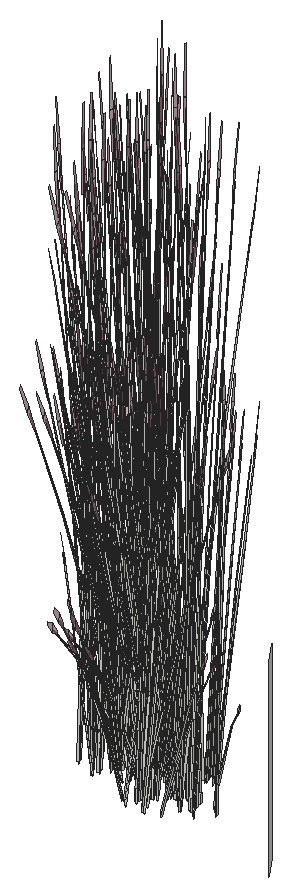
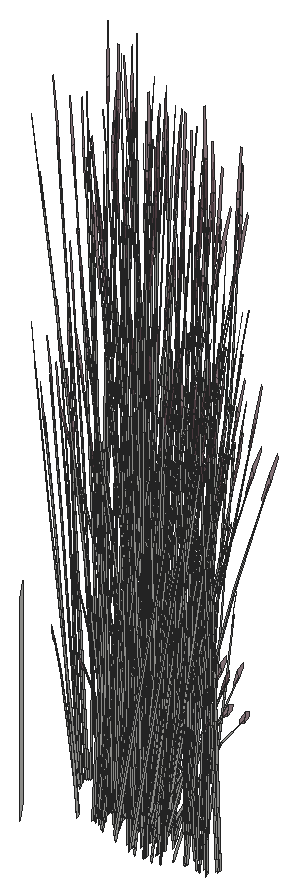
# SketchUp Ruby script. Lengths in inches.
U = 1.inch
M = Sketchup.active_model
def pt(a) = Geom::Point3d.new(a.map { |v| v * U })
def face(e, loops, mat)
  f = e.add_face(loops[0].map { |a| pt(a) })
  loops[1..].each { |l| e.add_face(l.map { |a| pt(a) }).erase! }
  f.material = f.back_material = mat if mat
  f
end
# faces: each face lists its corners as indices into pts; further lists are holes
def faces(e, pts, list, mat = nil) = list.each { |f| face(e, (f[0].is_a?(Array) ? f : [f]).map { |l| l.map { |i| pts[i] } }, mat) }
# xy, xz, yz: faces in a plane at the given z, y or x. An outline is a flat list of corners, or four numbers for a rectangle; further outlines are holes
def ring(l) = l.size == 4 ? [[l[0], l[1]], [l[2], l[1]], [l[2], l[3]], [l[0], l[3]]] : l.each_slice(2).to_a
def flat(e, list, mat, &to3) = list.each { |f| face(e, (f[0].is_a?(Array) ? f : [f]).map { |l| ring(l).map { |u, v| to3.(u, v) } }, mat) }
def xy(e, z, list, mat = nil) = flat(e, list, mat) { |x, y| [x, y, z] }
def xz(e, y, list, mat = nil) = flat(e, list, mat) { |x, z| [x, y, z] }
def yz(e, x, list, mat = nil) = flat(e, list, mat) { |y, z| [x, y, z] }
def lines(e, pts, list) = list.each { |a, b| e.add_line(pt(pts[a]), pt(pts[b])) }
# prism: a flat outline (further loops are holes) pulled along v
def prism(e, loops, v, mat = nil)
  f = face(e, loops, mat); d = Geom::Vector3d.new(v.map { |x| x * U })
  f.pushpull(f.normal.samedirection?(d) ? d.length : -d.length)
end
def box(e, o, s, mat = nil) = prism(e, [[o, [o[0] + s[0], o[1], o[2]], [o[0] + s[0], o[1] + s[1], o[2]], [o[0], o[1] + s[1], o[2]]]], [0, 0, s[2]], mat)
def at(x, y, z, deg = 0) = Geom::Transformation.translation(pt([x, y, z])) * Geom::Transformation.rotation(ORIGIN, Z_AXIS, deg.degrees)
def axes(o, x, y, z) = Geom::Transformation.new([*x, 0, *y, 0, *z, 0, *pt(o).to_a, 1])
def part(name) = M.definitions.add(name)
# library, detail: a bought-in or finely detailed component or shape, given as its bounding box
def library(name, o, s) = part(name).tap { |d| box(d.entities, o, s) }
def detail(e, o, s) = box(e.add_group.entities, o, s)
def put(e, d, t, mat = nil) = e.add_instance(d, t).tap { |i| i.material = mat if mat }
def group(e, t, mat = nil) = e.add_group.tap { |g| g.transformation = t; g.material = mat if mat }.entities
root = M.entities
M.materials.add("LightPink_Translucent").color = [144, 107, 117]
M.materials["LightPink_Translucent"].alpha = 0.75
c1 = part("blade")
p = [[2.15,0.21,22],[0,0.17,0],[0.09,0.45,0],[2.18,0.31,22],[2.29,0.31,22],[0.38,0.45,0],
  [2.48,0.24,33],[2.49,0.24,33],[2.48,0.22,33]]
faces(c1.entities,p,[[0,1,2,3],[4,5,2,3],[6,3,4,7],[8,0,3,6]])
c2 = part("seeds")
p = [[0.3,-0.1,1.38],[-0.01,-0.03,1.59],[-0.01,-0.03,0.03],[0.14,-0.07,-0.07],[0.29,-0.03,3],[0.15,0.01,3.11]]
faces(c2.entities,p,[[0,1,2,3],[1,0,4,5]],"LightPink_Translucent")
c3 = part("blade with seeds")
put(c3.entities,c1,at(0,0,0))
put(c3.entities,c2,axes([2.4,0.25,30.99],[1.5799,-0.05474,1.17369],[-0.12525,1.92788,0.29478],[-0.07173,-0.02425,1.56792]))
p = [[371.24,353.33,618],[372.76,351.04,618],[372.76,351.04,636],[371.24,353.33,636]]
faces(root,p,[[0,1,2,3]])
put(root,c3,axes([357.23,353.86,621.875],[0.1311,0.08035,1.71376],[-0.27131,0.33708,0.13857],[-0.16909,-0.15206,0.73262]))
put(root,c3,axes([354.31,353.96,620.02],[0,-0.46636,-0.49651],[0.39487,0,0],[0,-0.10622,1.57504]))
put(root,c3,axes([355.34,354.5,620.67],[-0.39748,-0.22252,-0.29095],[0.19139,-0.46966,-0.50002],[-0.01249,-0.11531,1.59708]))
put(root,c3,axes([357.2,353.12,622.72],[-0.07594,-0.00329,1.74944],[-0.24177,0.32918,-0.27667],[-0.129,-0.06726,0.14031]))
put(root,c3,axes([354.52,353.34,623.05],[-0.23881,0.24554,0.35414],[-0.22606,-0.28036,-0.4572],[0.0344,-0.14245,0.87481]))
put(root,c3,axes([353.38,354.22,620.67],[-0.04113,-0.53214,-0.29095],[0.42835,-0.03218,-0.50002],[0.07543,-0.07088,1.59708]))
put(root,c3,axes([354.48,353.97,620.03],[0.24637,-0.29097,-0.30978],[0.24637,0.29097,0.30978],[0,-0.09372,1.38974]))
put(root,c3,axes([355.59,352.09,620.13],[-0.2439,0.26754,-0.03893],[-0.22348,-0.29302,-0.17649],[-0.01573,-0.08303,0.58215]))
put(root,c3,axes([353.32,353.04,620.03],[0.32928,0.11539,-0.30978],[-0.08291,0.40636,0.30978],[0.06638,-0.04686,1.38974]))
put(root,c3,axes([353.25,352.85,620.02],[0.33032,-0.23318,-0.49651],[0.19744,0.41812,0],[0.07523,-0.05311,1.57504]))
put(root,c3,axes([357.15,353.87,623.09],[0.29147,-0.34417,0.53763],[0.25138,0.3655,0.4433],[-0.13675,-0.06349,1.11249]))
put(root,c3,axes([358.1,353.25,623.43],[-0.23555,0.44708,-0.13619],[-0.34112,-0.25757,-0.75594],[-0.11858,-0.12631,1.14864]))
put(root,c3,axes([358,353.61,622.98],[-0.30095,-0.22541,-0.71045],[0.21388,-0.395,0.08574],[-0.10904,-0.13459,1.00501]))
put(root,c3,axes([357.86,353.625,622.68],[-0.34827,0.11086,-0.51099],[-0.06092,-0.41983,-0.3958],[-0.09354,-0.12031,0.97773]))
put(root,c3,axes([355.38,354.15,620.21],[0.17124,-0.42022,-0.44739],[0.35581,0.20224,0.21531],[0,-0.09687,1.43643]))
put(root,c3,axes([354.74,353.11,622.73],[0.29004,0.02173,0.0643],[-0.00795,0.32812,0.50621],[0.03035,-0.12569,0.77189]))
put(root,c3,axes([353.64,353.81,620.06],[0.23773,-0.35053,-0.62353],[0.29532,0.31785,-0.16365],[0.09526,-0.08744,1.37633]))
put(root,c3,axes([357.41,353.24,619.49],[-0.03419,0.06144,1.76342],[-0.3455,0.13246,-0.26939],[-0.08346,-0.12049,0.30037]))
put(root,c3,axes([354.64,353.08,622.73],[0.25132,0.3182,0.48003],[-0.2669,0.27442,0.3958],[0.04636,-0.14929,0.9933]))
put(root,c3,axes([358.76,353.87,621.875],[0.1311,0.08035,1.71376],[-0.27131,0.33708,0.13857],[-0.16909,-0.15206,0.73262]))
put(root,c3,axes([359.77,350.87,621.34],[0.10032,-0.06746,1.77064],[0.0346,0.47103,0.13857],[-0.2173,0.0625,0.63284]))
put(root,c3,axes([354.93,354.1,623.05],[-0.30722,0.06665,0.35414],[-0.08112,-0.381,-0.4572],[0.08804,-0.10234,0.87481]))
put(root,c3,axes([358.69,351.18,622.72],[-0.05763,0.06055,1.74944],[0.0049,0.44239,-0.27667],[-0.13211,0.05753,0.14031]))
put(root,c3,axes([358.74,353.13,622.72],[-0.07594,-0.00329,1.74944],[-0.24177,0.32918,-0.27667],[-0.129,-0.06726,0.14031]))
put(root,c3,axes([355.09,354.13,623.03],[-0.32648,-0.25715,-0.1216],[0.18809,-0.3724,-0.67495],[0.09224,-0.12945,1.02557]))
put(root,c3,axes([358.88,350.93,622.53],[-0.29332,-0.1301,-0.35414],[0.08555,-0.37955,0.4572],[-0.11809,0.0348,0.87481]))
put(root,c3,axes([357.9,353.3125,622.53],[-0.05451,-0.37564,-0.35414],[0.31161,-0.09919,0.4572],[-0.0837,-0.10765,0.87481]))
put(root,c3,axes([355.1,352.65,620.375],[-0.22066,-0.46731,0],[0.36918,-0.26061,-0.51607],[0.08408,-0.05936,1.63711]))
put(root,c3,axes([359.08,351.125,622.68],[-0.09562,0.42421,-0.51099],[-0.32782,-0.1454,-0.3958],[-0.13199,0.0389,0.97773]))
put(root,c3,axes([354.94,352.84,619.49],[-0.05283,-0.03674,1.76342],[-0.13569,-0.41045,-0.26939],[0.09154,-0.11138,0.30037]))
put(root,c3,axes([358.92,351.1,619.49],[0.00895,0.0735,1.76342],[-0.18044,0.38382,-0.26939],[-0.12817,-0.01935,0.30037]))
put(root,c3,axes([358.08,353.62,623.05],[0.05451,0.37564,0.35414],[-0.31161,0.09919,-0.4572],[-0.0837,-0.10765,0.87481]))
put(root,c3,axes([354.93,353.83,622.68],[-0.09067,-0.42583,-0.51099],[0.34336,-0.07449,-0.3958],[0.0984,-0.11438,0.97773]))
put(root,c3,axes([358.72,356.16,621.33],[0.305,0.18805,1.51261],[-0.29879,0.40513,0.59816],[-0.13384,-0.24012,1.26806]))
put(root,c3,axes([358.68,353.88,623.09],[0.29147,-0.34417,0.53763],[0.25138,0.3655,0.4433],[-0.13675,-0.06349,1.11249]))
put(root,c3,axes([357.56,352.75,620.77],[0.18411,0.16231,1.1486],[-0.26813,0.09757,0.84392],[-0.05737,-0.12474,0.25299]))
put(root,c3,axes([358.95,350.89,622.73],[0.09971,-0.42522,0.48003],[0.32782,0.1454,0.3958],[-0.12892,0.02555,0.9933]))
put(root,c3,axes([359.0625,350.76,623.03],[0.17758,0.42229,-0.1216],[-0.31518,0.20752,-0.67495],[-0.13282,0.05572,1.02557]))
put(root,c3,axes([358.92,350.77,622.73],[-0.12963,-0.31798,0.0643],[0.23638,-0.15564,0.50621],[-0.1042,0.03071,0.77189]))
put(root,c3,axes([356.68,353.0625,623.05],[-0.23881,0.24554,0.35414],[-0.22606,-0.28036,-0.4572],[0.0344,-0.14245,0.87481]))
put(root,c3,axes([355.35,352.98,620.77],[-0.11756,0.2374,1.1486],[-0.10105,-0.31895,0.84392],[0.09709,-0.07992,0.25299]))
put(root,c3,axes([355.54,353.94,620.67],[-0.04113,-0.53214,-0.29095],[0.42835,-0.03218,-0.50002],[0.07543,-0.07088,1.59708]))
put(root,c3,axes([358.03,353.28,622.73],[0.16041,-0.29625,0.0643],[0.22843,0.17248,0.50621],[-0.07385,-0.09498,0.77189]))
put(root,c3,axes([359.64,353.26,623.43],[-0.23555,0.44708,-0.13619],[-0.34112,-0.25757,-0.75594],[-0.11858,-0.12631,1.14864]))
put(root,c3,axes([355.48,352.76,620.03],[0.32928,0.11539,-0.30978],[-0.08291,0.40636,0.30978],[0.06638,-0.04686,1.38974]))
put(root,c3,axes([359.54,353.625,622.98],[-0.30095,-0.22541,-0.71045],[0.21388,-0.395,0.08574],[-0.10904,-0.13459,1.00501]))
put(root,c3,axes([355.9,354.02,622.71],[-0.0461,-0.00354,1.77383],[-0.19143,-0.37951,-0.16761],[0.07688,-0.12478,0.31391]))
put(root,c3,axes([359.4,353.64,622.68],[-0.34827,0.11086,-0.51099],[-0.06092,-0.41983,-0.3958],[-0.09354,-0.12031,0.97773]))
put(root,c3,axes([357.125,354.86,620.02],[0,-0.46636,-0.49651],[0.39487,0,0],[0,-0.10622,1.57504]))
put(root,c3,axes([355.18,353.87,622.53],[0.30722,-0.06665,-0.35414],[0.08112,0.381,0.4572],[0.08804,-0.10234,0.87481]))
put(root,c3,axes([354.94,354,622.98],[0.18436,-0.36797,-0.71045],[0.32306,0.26151,0.08574],[0.11008,-0.13332,1.00501]))
put(root,c3,axes([355.4,352.58,620.02],[0.33032,-0.23318,-0.49651],[0.19744,0.41812,0],[0.07523,-0.05311,1.57504]))
put(root,c3,axes([358.95,353.25,619.49],[-0.03419,0.06144,1.76342],[-0.3455,0.13246,-0.26939],[-0.08346,-0.12049,0.30037]))
put(root,c3,axes([359.1875,350.89,623.05],[0.29332,0.1301,0.35414],[-0.08555,0.37955,-0.4572],[-0.11809,0.0348,0.87481]))
put(root,c3,axes([357.98,354.93,620.1],[-0.14494,-0.47823,-0.69835],[0.41752,-0.17223,-0.18329],[-0.01602,-0.16194,1.54149]))
put(root,c3,axes([358.93,353.41,623.03],[-0.34538,0.21713,-0.1216],[-0.16972,-0.38536,-0.67495],[-0.04557,-0.16239,1.02557]))
put(root,c3,axes([358.41,352.99,620.13],[-0.2439,0.26754,-0.03893],[-0.22348,-0.29302,-0.17649],[-0.01573,-0.08303,0.58215]))
put(root,c3,axes([355.21,353.66,620.59],[-0.12609,-0.01381,1.43002],[-0.12917,-0.37055,-0.30754],[0.1549,-0.10482,0.61141]))
put(root,c3,axes([359.61,352.66,620.02],[-0.33032,-0.23318,-0.49651],[0.19744,-0.41812,0],[-0.07523,-0.05311,1.57504]))
put(root,c3,axes([359.81,352.94,620.375],[-0.22066,0.46731,0],[-0.36918,-0.26061,-0.51607],[-0.08408,-0.05936,1.63711]))
put(root,c3,axes([359.43,353.33,622.53],[-0.05451,-0.37564,-0.35414],[0.31161,-0.09919,0.4572],[-0.0837,-0.10765,0.87481]))
put(root,c3,axes([355.8,353.54,620.06],[0.23773,-0.35053,-0.62353],[0.29532,0.31785,-0.16365],[0.09526,-0.08744,1.37633]))
put(root,c3,axes([358.83,353.5625,623.05],[-0.1064,0.35863,0.35414],[-0.31043,-0.1046,-0.4572],[-0.02846,-0.14439,0.87481]))
put(root,c3,axes([359.62,353.63,623.05],[0.05451,0.37564,0.35414],[-0.31161,0.09919,-0.4572],[-0.0837,-0.10765,0.87481]))
put(root,c3,axes([360.26,356.17,621.33],[0.305,0.18805,1.51261],[-0.29879,0.40513,0.59816],[-0.13384,-0.24012,1.26806]))
put(root,c3,axes([357.09,353.82,623.05],[-0.30722,0.06665,0.35414],[-0.08112,-0.381,-0.4572],[0.08804,-0.10234,0.87481]))
put(root,c3,axes([359.09,352.76,620.77],[0.18411,0.16231,1.1486],[-0.26813,0.09757,0.84392],[-0.05737,-0.12474,0.25299]))
put(root,c3,axes([360.51,351.84,620.67],[-0.35635,0.30962,-0.29095],[-0.23697,-0.43749,-0.50002],[-0.08792,-0.04443,1.59708]))
put(root,c3,axes([359.71,352.48,620.03],[-0.08291,-0.40636,-0.30978],[0.32928,-0.11539,0.30978],[-0.06638,-0.04686,1.38974]))
put(root,c3,axes([357.25,353.86,623.03],[-0.32648,-0.25715,-0.1216],[0.18809,-0.3724,-0.67495],[0.09224,-0.12945,1.02557]))
put(root,c3,axes([359.57,353.29,622.73],[0.16041,-0.29625,0.0643],[0.22843,0.17248,0.50621],[-0.07385,-0.09498,0.77189]))
put(root,c3,axes([358.66,354.875,620.02],[0,-0.46636,-0.49651],[0.39487,0,0],[0,-0.10622,1.57504]))
put(root,c3,axes([360.91,351.98,620.46],[-0.34464,-0.37536,-0.25192],[0.29,-0.42149,0.5513],[-0.0928,0.04391,1.68216]))
put(root,c3,axes([357.09,353.55,622.68],[-0.09067,-0.42583,-0.51099],[0.34336,-0.07449,-0.3958],[0.0984,-0.11438,0.97773]))
put(root,c3,axes([358.92,353.24,622.73],[0.26007,-0.1585,0.0643],[0.12729,0.28902,0.50621],[-0.02512,-0.1274,0.77189]))
put(root,c3,axes([362.62,352.39,621.875],[0.14639,-0.01056,1.71376],[-0.09712,0.45778,0.13857],[-0.20862,-0.02831,0.73262]))
put(root,c3,axes([357.51,352.7,620.77],[-0.11756,0.2374,1.1486],[-0.10105,-0.31895,0.84392],[0.09709,-0.07992,0.25299]))
put(root,c3,axes([360.01,352.7,620.48],[0.33032,0.23318,0.49651],[-0.19744,0.41812,0],[-0.07523,-0.05311,1.57504]))
put(root,c3,axes([357.37,353.76,622.73],[0.2423,0.19613,0.0643],[-0.14107,0.2793,0.50621],[0.07768,-0.0903,0.77189]))
put(root,c3,axes([359.52,354.94,620.1],[-0.14494,-0.47823,-0.69835],[0.41752,-0.17223,-0.18329],[-0.01602,-0.16194,1.54149]))
put(root,c3,axes([360.47,353.42,623.03],[-0.34538,0.21713,-0.1216],[-0.16972,-0.38536,-0.67495],[-0.04557,-0.16239,1.02557]))
put(root,c3,axes([357.3,353.68,622.73],[0.08753,0.42921,0.48003],[-0.34336,0.07449,0.3958],[0.1012,-0.10094,0.9933]))
put(root,c3,axes([357.92,353.55,620.375],[-0.22066,-0.46731,0],[0.36918,-0.26061,-0.51607],[0.08408,-0.05936,1.63711]))
put(root,c3,axes([360.48,351.97,620.62],[-0.06809,0.4162,0.1448],[-0.33266,-0.07225,-0.41347],[-0.06054,-0.04274,1.26744]))
put(root,c3,axes([359.94,353,620.13],[-0.2439,0.26754,-0.03893],[-0.22348,-0.29302,-0.17649],[-0.01573,-0.08303,0.58215]))
put(root,c3,axes([358.05,353.74,622.71],[-0.0461,-0.00354,1.77383],[-0.19143,-0.37951,-0.16761],[0.07688,-0.12478,0.31391]))
put(root,c3,axes([357.34,353.6,622.53],[0.30722,-0.06665,-0.35414],[0.08112,0.381,0.4572],[0.08804,-0.10234,0.87481]))
put(root,c3,axes([357.1,353.72,622.98],[0.18436,-0.36797,-0.71045],[0.32306,0.26151,0.08574],[0.11008,-0.13332,1.00501]))
put(root,c3,axes([359.65,353.9,623.03],[-0.3879,-0.02311,-0.1216],[0.0106,-0.43749,-0.67495],[0.02694,-0.1685,1.02557]))
put(root,c3,axes([360.36,353.57,623.05],[-0.1064,0.35863,0.35414],[-0.31043,-0.1046,-0.4572],[-0.02846,-0.14439,0.87481]))
put(root,c3,axes([359.5,353.96,623.05],[-0.23881,0.24554,0.35414],[-0.22606,-0.28036,-0.4572],[0.0344,-0.14245,0.87481]))
put(root,c3,axes([360.37,351.57,620.36],[0.44609,0.09826,0.45755],[-0.09078,0.55493,0.17955],[-0.06519,-0.05359,1.58856]))
put(root,c3,axes([363.0625,351.97,622.98],[-0.35281,-0.01123,-0.71045],[0.0237,-0.47284,0.08574],[-0.14947,-0.0499,1.00501]))
put(root,c3,axes([362.78,352.08,620.59],[0.06891,0.12984,1.43002],[-0.15879,0.35293,-0.30754],[-0.16304,-0.08436,0.61141]))
put(root,c3,axes([357.36,353.39,620.59],[-0.12609,-0.01381,1.43002],[-0.12917,-0.37055,-0.30754],[0.1549,-0.10482,0.61141]))
put(root,c3,axes([360.13,352.46,620.47],[0.37926,-0.12378,0.17642],[0.09365,0.46065,0.35086],[-0.03382,-0.06712,1.60407]))
put(root,c3,axes([358.22,353.48,620.02],[0.33032,-0.23318,-0.49651],[0.19744,0.41812,0],[0.07523,-0.05311,1.57504]))
put(root,c3,axes([360.62,352.53,620.2],[-0.35581,-0.20937,0],[0.17124,-0.43505,0],[0,0,1.62707]))
put(root,c3,axes([362.94,352.0625,622.68],[-0.25628,0.30892,-0.51099],[-0.22444,-0.32634,-0.3958],[-0.13021,-0.047,0.97773]))
put(root,c3,axes([362.58,351.2,622.71],[0.02617,0.04654,1.77383],[-0.12614,0.41836,-0.16761],[-0.12775,0.00303,0.31391]))
put(root,c3,axes([361.26,352.49,620.47],[0.10196,-0.46348,0.17642],[0.3731,0.13116,0.35086],[-0.06445,0.00226,1.60407]))
put(root,c3,axes([361.08,351.67,620.72],[0.38326,-0.02879,0.44739],[0.03466,0.47788,-0.21531],[-0.06861,0.04843,1.43643]))
put(root,c3,axes([360.46,353.25,622.73],[0.26007,-0.1585,0.0643],[0.12729,0.28902,0.50621],[-0.02512,-0.1274,0.77189]))
put(root,c3,axes([362.5625,352.74,622.73],[0.09971,-0.42522,0.48003],[0.32782,0.1454,0.3958],[-0.12892,0.02555,0.9933]))
put(root,c3,axes([360.37,353.28,622.73],[0.34777,0.12192,0.48003],[-0.11892,0.40083,0.3958],[-0.0209,-0.15763,0.9933]))
put(root,c3,axes([363.08,351.74,623.03],[-0.0189,0.47427,-0.1216],[-0.35781,-0.01296,-0.67495],[-0.13781,-0.03295,1.02557]))
put(root,c3,axes([358.23,354.2,622.72],[0.04898,-0.07104,1.74944],[-0.06269,-0.43574,-0.27667],[0.12289,-0.08262,0.14031]))
put(root,c3,axes([360.7,352.35,620.2],[-0.11516,-0.40207,0],[0.32884,-0.1408,0],[0,0,1.54371]))
put(root,c3,axes([359.62,353.62,622.53],[0.23881,-0.24554,-0.35414],[0.22606,0.28036,0.4572],[0.0344,-0.14245,0.87481]))
put(root,c3,axes([362.37,352.47,620.77],[0.22533,-0.03337,1.1486],[-0.14293,0.29403,0.84392],[-0.11135,-0.04411,0.25299]))
put(root,c3,axes([359.71,353.74,622.73],[0.29004,0.02173,0.0643],[-0.00795,0.32812,0.50621],[0.03035,-0.12569,0.77189]))
put(root,c3,axes([359.46,353.57,620.375],[-0.22066,-0.46731,0],[0.36918,-0.26061,-0.51607],[0.08408,-0.05936,1.63711]))
put(root,c3,axes([358.62,354.4375,620.06],[0.23773,-0.35053,-0.62353],[0.29532,0.31785,-0.16365],[0.09526,-0.08744,1.37633]))
put(root,c3,axes([359.62,353.71,622.73],[0.25132,0.3182,0.48003],[-0.2669,0.27442,0.3958],[0.04636,-0.14929,0.9933]))
put(root,c3,axes([361.84,351.3,620.47],[-0.2773,-0.3397,0.17642],[0.27945,-0.32949,0.35086],[-0.03063,0.06937,1.60407]))
put(root,c3,axes([361.1,351.32,620.29],[0,0.53934,-0.05637],[-0.44133,0,0],[0,0.01695,1.79368]))
put(root,c3,axes([361.18,353.91,623.03],[-0.3879,-0.02311,-0.1216],[0.0106,-0.43749,-0.67495],[0.02694,-0.1685,1.02557]))
put(root,c3,axes([363.71,353.62,620.06],[-0.36714,-0.07646,-0.62353],[0.07747,-0.47163,-0.16365],[-0.10956,-0.05715,1.37633]))
put(root,c3,axes([361.03,353.98,623.05],[-0.23881,0.24554,0.35414],[-0.22606,-0.28036,-0.4572],[0.0344,-0.14245,0.87481]))
put(root,c3,axes([363.13,351.93,623.05],[0.20082,0.29199,0.35414],[-0.2293,0.2764,-0.4572],[-0.1165,-0.04206,0.87481]))
put(root,c3,axes([360.07,354.76,623.03],[-0.32648,-0.25715,-0.1216],[0.18809,-0.3724,-0.67495],[0.09224,-0.12945,1.02557]))
put(root,c3,axes([361.29,350.1,620.47],[-0.37926,0.12378,0.17642],[-0.09365,-0.46065,0.35086],[0.03382,0.06712,1.60407]))
put(root,c3,axes([359.92,353.47,619.49],[-0.05283,-0.03674,1.76342],[-0.13569,-0.41045,-0.26939],[0.09154,-0.11138,0.30037]))
put(root,c3,axes([361.17,351.43,620.21],[0.24637,0.30123,0],[-0.24637,0.30123,0],[0,0,1.69266]))
put(root,c3,axes([361.17,351.08,620.72],[0.17124,-0.42022,0.44739],[0.35581,0.20224,-0.21531],[0,0.09687,1.43643]))
put(root,c3,axes([361.05,350.98,620.38],[-0.44609,-0.09826,0.49198],[0.09078,-0.55493,0.19306],[0.06519,0.05359,1.70813]))
put(root,c3,axes([359.91,354.45,622.68],[-0.09067,-0.42583,-0.51099],[0.34336,-0.07449,-0.3958],[0.0984,-0.11438,0.97773]))
put(root,c3,axes([359.76,353.49,620.02],[0.33032,-0.23318,-0.49651],[0.19744,0.41812,0],[0.07523,-0.05311,1.57504]))
put(root,c3,axes([361.18,351.23,620.21],[0.39487,0,0],[0,0.48281,0],[0,0,1.78407]))
put(root,c3,axes([360.8,350.7,620.72],[-0.21202,-0.39143,0.44739],[0.32115,-0.27564,-0.21531],[0.06861,0.04843,1.43643]))
put(root,c3,axes([361.32,351.18,620.62],[0.32884,-0.136,0.1448],[0.11516,0.38837,-0.41347],[0,0.08547,1.26744]))
put(root,c3,axes([360.33,353.61,620.77],[-0.11756,0.2374,1.1486],[-0.10105,-0.31895,0.84392],[0.09709,-0.07992,0.25299]))
put(root,c3,axes([362.7,353.01,620.375],[-0.44133,0,0],[0,-0.52122,-0.51607],[0,-0.11871,1.63711]))
put(root,c3,axes([362.07,351.32,620.48],[0,-0.46636,0.49651],[0.39487,0,0],[0,0.10622,1.57504]))
put(root,c3,axes([360.875,354.65,622.71],[-0.0461,-0.00354,1.77383],[-0.19143,-0.37951,-0.16761],[0.07688,-0.12478,0.31391]))
put(root,c3,axes([361.16,353.63,622.53],[0.23881,-0.24554,-0.35414],[0.22606,0.28036,0.4572],[0.0344,-0.14245,0.87481]))
put(root,c3,axes([360.94,350.59,620.62],[0.06809,-0.4162,0.1448],[0.33266,0.07225,-0.41347],[0.06054,0.04274,1.26744]))
put(root,c3,axes([361.25,353.75,622.73],[0.29004,0.02173,0.0643],[-0.00795,0.32812,0.50621],[0.03035,-0.12569,0.77189]))
put(root,c3,axes([360.16,354.5,622.53],[0.30722,-0.06665,-0.35414],[0.08112,0.381,0.4572],[0.08804,-0.10234,0.87481]))
put(root,c3,axes([359.92,354.625,622.98],[0.18436,-0.36797,-0.71045],[0.32306,0.26151,0.08574],[0.11008,-0.13332,1.00501]))
put(root,c3,axes([360.15,354.45,620.06],[0.23773,-0.35053,-0.62353],[0.29532,0.31785,-0.16365],[0.09526,-0.08744,1.37633]))
put(root,c3,axes([363.04,352.875,620.33],[-0.32829,0.39208,0.30756],[-0.32849,-0.38796,-0.36492],[-0.01146,-0.11134,1.64885]))
put(root,c3,axes([361.16,353.72,622.73],[0.25132,0.3182,0.48003],[-0.2669,0.27442,0.3958],[0.04636,-0.14929,0.9933]))
put(root,c3,axes([363.9,353.47,620.21],[-0.21202,-0.39143,-0.44739],[0.32115,-0.27564,0.21531],[-0.06861,-0.04843,1.43643]))
put(root,c3,axes([361.13,352.3,620.18],[0.37054,-0.15823,-0.19198],[0.1302,0.45581,0.00008],[0.0409,-0.01749,1.73897]))
put(root,c3,axes([361.14,350.94,620.21],[0.21202,0.39143,-0.44739],[-0.32115,0.27564,0.21531],[0.06861,0.04843,1.43643]))
put(root,c3,axes([363.93,353.69,620.4375],[0.09355,-0.55261,-0.23429],[0.44354,0.09633,0.51271],[-0.0775,-0.07631,1.5644]))
put(root,c3,axes([360.18,354.29,620.59],[-0.12609,-0.01381,1.43002],[-0.12917,-0.37055,-0.30754],[0.1549,-0.10482,0.61141]))
put(root,c3,axes([361.61,354.77,623.03],[-0.32648,-0.25715,-0.1216],[0.18809,-0.3724,-0.67495],[0.09224,-0.12945,1.02557]))
put(root,c3,axes([362.97,353.09,620.48],[0,0.46636,0.49651],[-0.39487,0,0],[0,-0.10622,1.57504]))
put(root,c3,axes([361.72,350.07,620.03],[0.08291,0.40636,-0.30978],[-0.32928,0.11539,0.30978],[0.06638,0.04686,1.38974]))
put(root,c3,axes([361.45,353.48,619.49],[-0.05283,-0.03674,1.76342],[-0.13569,-0.41045,-0.26939],[0.09154,-0.11138,0.30037]))
put(root,c3,axes([360.91,350.72,620.67],[0.35635,-0.30962,-0.29095],[0.23697,0.43749,-0.50002],[0.08792,0.04443,1.59708]))
put(root,c3,axes([363.83,353.2,620.67],[-0.39748,-0.22252,-0.29095],[0.19139,-0.46966,-0.50002],[-0.01249,-0.11531,1.59708]))
put(root,c3,axes([361.44,354.47,622.68],[-0.09067,-0.42583,-0.51099],[0.34336,-0.07449,-0.3958],[0.0984,-0.11438,0.97773]))
put(root,c3,axes([360.01,350.44,619.59],[-0.3474,0.18671,1.28929],[-0.11057,-0.53572,0.50096],[0.21332,0.00891,1.46642]))
put(root,c3,axes([361.87,353.62,620.77],[-0.11756,0.2374,1.1486],[-0.10105,-0.31895,0.84392],[0.09709,-0.07992,0.25299]))
put(root,c3,axes([363.87,353.33,620.72],[-0.17124,0.42022,0.44739],[-0.35581,-0.20224,-0.21531],[0,-0.09687,1.43643]))
put(root,c3,axes([361.81,349.9,620.02],[0.33032,0.23318,-0.49651],[-0.19744,0.41812,0],[0.07523,0.05311,1.57504]))
put(root,c3,axes([362.41,354.66,622.71],[-0.0461,-0.00354,1.77383],[-0.19143,-0.37951,-0.16761],[0.07688,-0.12478,0.31391]))
put(root,c3,axes([362.57,352.6,621.93],[-0.06755,-0.39203,-0.03492],[0.31928,-0.09013,-0.15832],[0.06667,0.02485,0.52218]))
put(root,c3,axes([361.7,354.51,622.53],[0.30722,-0.06665,-0.35414],[0.08112,0.381,0.4572],[0.08804,-0.10234,0.87481]))
put(root,c3,axes([361.45,354.64,622.98],[0.18436,-0.36797,-0.71045],[0.32306,0.26151,0.08574],[0.11008,-0.13332,1.00501]))
put(root,c3,axes([361.33,350.79,620.06],[0.36714,0.07646,-0.62353],[-0.07747,0.47163,-0.16365],[0.10956,0.05715,1.37633]))
put(root,c3,axes([364.61,353.38,620.3],[-0.32829,-0.4014,-0.06131],[0.32849,-0.40164,0],[-0.01146,-0.01402,1.75571]))
put(root,c3,axes([363.95,352.92,620.36],[0.15345,0.52148,0.45755],[-0.43845,0.18134,0.17955],[0.00536,-0.09582,1.58856]))
put(root,c3,axes([362.28,351.7,622.73],[0.12963,0.31798,0.0643],[-0.23638,0.15564,0.50621],[0.1042,-0.03071,0.77189]))
put(root,c3,axes([361.72,354.3,620.59],[-0.12609,-0.01381,1.43002],[-0.12917,-0.37055,-0.30754],[0.1549,-0.10482,0.61141]))
put(root,c3,axes([361.74,352.58,623.03],[0.0189,-0.47427,-0.1216],[0.35781,0.01296,-0.67495],[0.13781,0.03295,1.02557]))
put(root,c3,axes([362.26,351.58,622.73],[-0.09971,0.42522,0.48003],[-0.32782,-0.1454,0.3958],[0.12892,-0.02555,0.9933]))
put(root,c3,axes([364.5,352.96,620.21],[0,-0.53961,0],[0.44133,0,0],[0,0,1.79456]))
put(root,c3,axes([364.09,353.06,620.43],[0.39767,0.22603,0.24065],[-0.19139,0.46966,0.50002],[0,-0.10827,1.60543]))
put(root,c3,axes([363.96,352.74,620.72],[-0.38326,0.02879,0.44739],[-0.03466,-0.47788,-0.21531],[0.06861,-0.04843,1.43643]))
put(root,c3,axes([363.78,351.92,620.47],[-0.10196,0.46348,0.17642],[-0.3731,-0.13116,0.35086],[0.06445,-0.00226,1.60407]))
put(root,c3,axes([362.95,351.61,620.77],[-0.21807,0.07699,1.1486],[0.10265,-0.31819,0.84392],[0.11568,0.02177,0.25299]))
put(root,c3,axes([362.33,351.54,622.53],[0.29332,0.1301,-0.35414],[-0.08555,0.37955,0.4572],[0.11809,-0.0348,0.87481]))
put(root,c3,axes([362.72,351.17,619.49],[-0.01845,-0.0708,1.76342],[0.12793,-0.41416,-0.26939],[0.12905,-0.00596,0.30037]))
put(root,c3,axes([364.29,352.62,620.36],[-0.29264,0.42323,0.45755],[-0.34767,-0.3736,0.17955],[0.07055,-0.04224,1.58856]))
put(root,c3,axes([362.85,352.96,622.71],[-0.03191,-0.04083,1.77383],[0.06981,-0.43764,-0.16761],[0.12571,-0.02796,0.31391]))
put(root,c3,axes([361.53,351.07,621.875],[-0.14639,0.01056,1.71376],[0.09712,-0.45778,0.13857],[0.20862,0.02831,0.73262]))
put(root,c3,axes([363.97,351.46,620.03],[0.32928,0.11539,-0.30978],[-0.08291,0.40636,0.30978],[0.06638,-0.04686,1.38974]))
put(root,c3,axes([364.56,352.4375,620.62],[0.06809,-0.4162,0.1448],[0.33266,0.07225,-0.41347],[0.06054,0.04274,1.26744]))
put(root,c3,axes([365.03,351.71,620.48],[-0.33032,-0.23318,0.49651],[0.19744,-0.41812,0],[0.07523,0.05311,1.57504]))
put(root,c3,axes([365.58,352.52,623.05],[-0.30722,0.06665,0.35414],[-0.08112,-0.381,-0.4572],[0.08804,-0.10234,0.87481]))
put(root,c3,axes([363.625,352.3,619.59],[-0.3474,0.18671,1.28929],[-0.11057,-0.53572,0.50096],[0.21332,0.00891,1.46642]))
put(root,c3,axes([365.22,351.47,620.375],[0.22066,-0.46731,0],[0.36918,0.26061,-0.51607],[0.08408,0.05936,1.63711]))
put(root,c3,axes([365.63,353.43,623.05],[-0.29332,-0.1301,0.35414],[0.08555,-0.37955,-0.4572],[0.11809,-0.0348,0.87481]))
put(root,c3,axes([366.5,352.92,620.26],[-0.21881,-0.29821,-0.06488],[0.23965,-0.27324,-0.29416],[0.0679,-0.01924,0.97024]))
put(root,c3,axes([365.86,352.46,622.73],[0.2423,0.19613,0.0643],[-0.14107,0.2793,0.50621],[0.07768,-0.0903,0.77189]))
put(root,c3,axes([365.79,352.38,622.73],[0.08753,0.42921,0.48003],[-0.34336,0.07449,0.3958],[0.1012,-0.10094,0.9933]))
put(root,c3,axes([365.76,353.56,623.03],[-0.17758,-0.42229,-0.1216],[0.31518,-0.20752,-0.67495],[0.13282,-0.05572,1.02557]))
put(root,c3,axes([365.74,353.2,622.68],[0.09562,-0.42421,-0.51099],[0.32782,0.1454,-0.3958],[0.13199,-0.0389,0.97773]))
put(root,c3,axes([366.09,353.32,619.98],[-0.22732,0.05597,1.41583],[-0.03618,-0.44548,0.08104],[0.15921,-0.06743,0.80566]))
put(root,c3,axes([365.68,353.35,622.98],[0.31014,-0.20596,-0.71045],[0.17284,0.42397,0.08574],[0.14985,-0.04816,1.00501]))
put(root,c3,axes([366.72,352.9,622.72],[0.04898,-0.07104,1.74944],[-0.06269,-0.43574,-0.27667],[0.12289,-0.08262,0.14031]))
